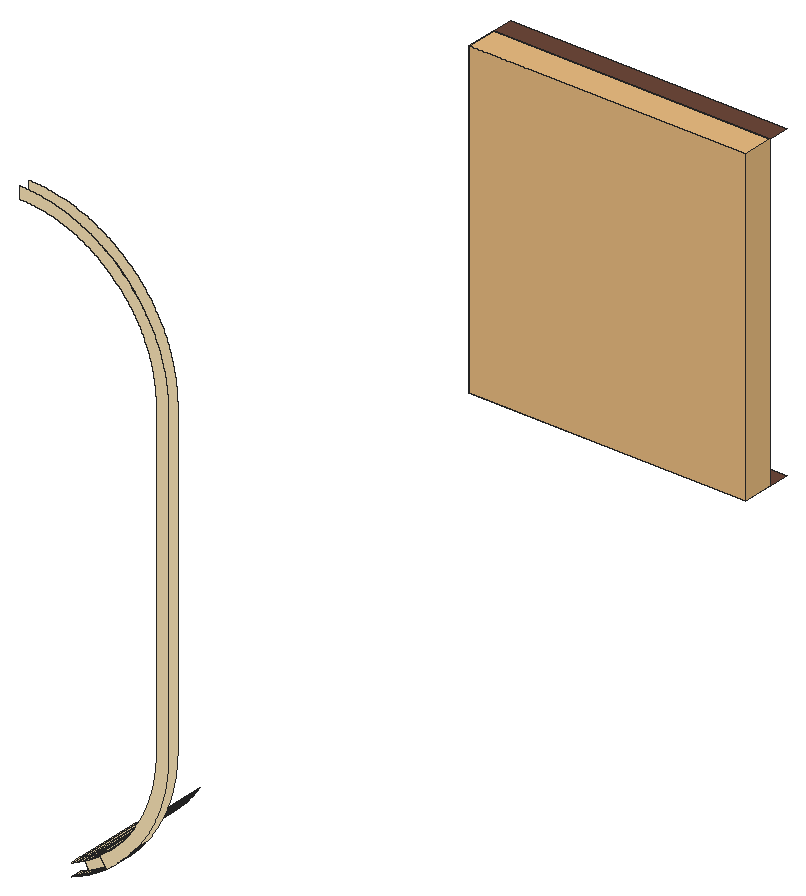
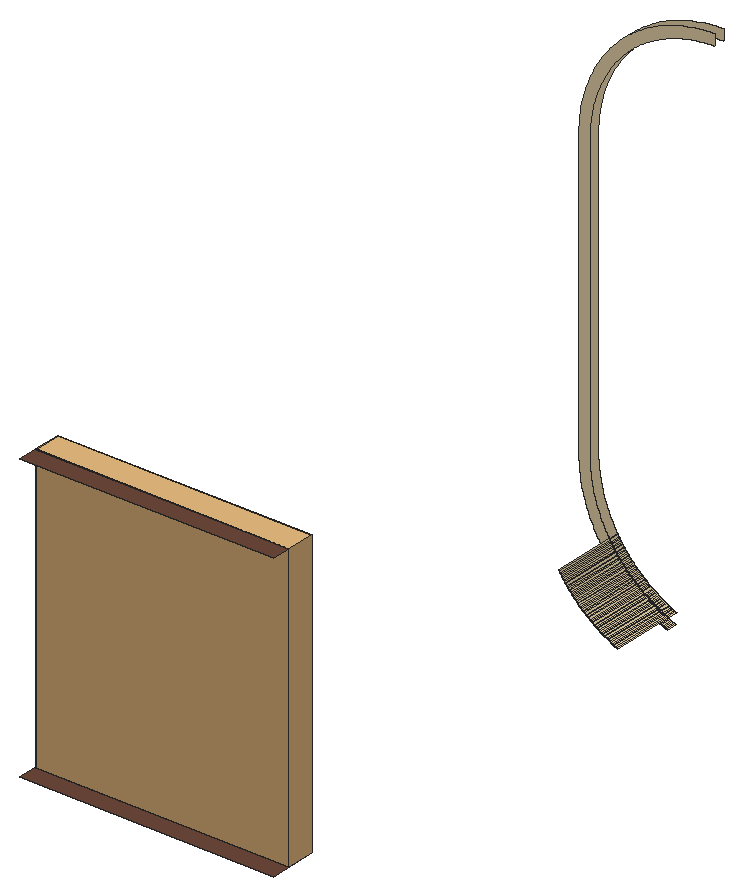
# SketchUp Ruby script. Lengths in inches.
U = 1.inch
M = Sketchup.active_model
def pt(a) = Geom::Point3d.new(a.map { |v| v * U })
def face(e, loops, mat)
  f = e.add_face(loops[0].map { |a| pt(a) })
  loops[1..].each { |l| e.add_face(l.map { |a| pt(a) }).erase! }
  f.material = f.back_material = mat if mat
  f
end
# faces: each face lists its corners as indices into pts; further lists are holes
def faces(e, pts, list, mat = nil) = list.each { |f| face(e, (f[0].is_a?(Array) ? f : [f]).map { |l| l.map { |i| pts[i] } }, mat) }
# xy, xz, yz: faces in a plane at the given z, y or x. An outline is a flat list of corners, or four numbers for a rectangle; further outlines are holes
def ring(l) = l.size == 4 ? [[l[0], l[1]], [l[2], l[1]], [l[2], l[3]], [l[0], l[3]]] : l.each_slice(2).to_a
def flat(e, list, mat, &to3) = list.each { |f| face(e, (f[0].is_a?(Array) ? f : [f]).map { |l| ring(l).map { |u, v| to3.(u, v) } }, mat) }
def xy(e, z, list, mat = nil) = flat(e, list, mat) { |x, y| [x, y, z] }
def xz(e, y, list, mat = nil) = flat(e, list, mat) { |x, z| [x, y, z] }
def yz(e, x, list, mat = nil) = flat(e, list, mat) { |y, z| [x, y, z] }
def lines(e, pts, list) = list.each { |a, b| e.add_line(pt(pts[a]), pt(pts[b])) }
# prism: a flat outline (further loops are holes) pulled along v
def prism(e, loops, v, mat = nil)
  f = face(e, loops, mat); d = Geom::Vector3d.new(v.map { |x| x * U })
  f.pushpull(f.normal.samedirection?(d) ? d.length : -d.length)
end
def box(e, o, s, mat = nil) = prism(e, [[o, [o[0] + s[0], o[1], o[2]], [o[0] + s[0], o[1] + s[1], o[2]], [o[0], o[1] + s[1], o[2]]]], [0, 0, s[2]], mat)
def at(x, y, z, deg = 0) = Geom::Transformation.translation(pt([x, y, z])) * Geom::Transformation.rotation(ORIGIN, Z_AXIS, deg.degrees)
def axes(o, x, y, z) = Geom::Transformation.new([*x, 0, *y, 0, *z, 0, *pt(o).to_a, 1])
def part(name) = M.definitions.add(name)
# library, detail: a bought-in or finely detailed component or shape, given as its bounding box
def library(name, o, s) = part(name).tap { |d| box(d.entities, o, s) }
def detail(e, o, s) = box(e.add_group.entities, o, s)
def put(e, d, t, mat = nil) = e.add_instance(d, t).tap { |i| i.material = mat if mat }
def group(e, t, mat = nil) = e.add_group.tap { |g| g.transformation = t; g.material = mat if mat }.entities
root = M.entities
M.materials.add("1026 AP 7946 SUNNY SIDE UP").color = [254, 231, 186]
M.materials.add("1916 AP K226 Macadamia Cream-N").color = [109, 72, 58]
c1 = library("Glazed double door",[0,0,0],[5.31,78.43,99.16])
xy(root,162,[[141,326,189,335]],"1916 AP K226 Macadamia Cream-N")
xy(root,216,[[141,326,189,335]],"1916 AP K226 Macadamia Cream-N")
xz(root,213.1,[[168.28,146.97,168.49,147.12,168.69,147.27,168.9,147.42,169.3,147.74,169.49,147.9,169.69,148.06,169.89,148.23,170.08,148.4,170.27,148.56,170.46,148.74,170.84,149.08,171.02,149.26,171.2,149.4375,171.38,149.62,171.5625,149.8,171.74,149.98,171.92,150.16,172.26,150.54,172.44,150.73,172.6,150.92,172.77,151.11,172.94,151.31,173.1,151.51,173.26,151.7,173.58,152.1,173.73,152.31,173.88,152.51,174.03,152.72,174.18,152.92,174.48,153.34,174.62,153.56,174.9,153.98,175.03,154.2,175.17,154.42,175.3,154.63,175.56,155.07,175.68,155.3,175.81,155.52,175.93,155.74,176.17,156.2,176.28,156.42,176.61,157.11,176.72,157.35,176.92,157.81,177.12,158.29,177.21,158.52,177.48,159.24,177.56,159.48,177.65,159.72,177.73,159.97,177.81,160.21,177.88,160.45,177.95,160.7,178.02,160.94,178.09,161.1875,178.16,161.44,178.22,161.68,178.4,162.43,178.6,163.43,178.68,163.93,178.72,164.19,178.75,164.4375,178.79,164.69,178.82,164.94,178.85,165.2,178.875,165.45,178.9,165.71,178.92,165.96,178.9375,166.21,178.95,166.47,178.97,166.72,178.98,166.98,178.99,167.23,179,167.49,179,222.51,178.99,222.77,178.98,223.02,178.97,223.28,178.95,223.53,178.9375,223.79,178.92,224.04,178.9,224.29,178.875,224.55,178.85,224.8,178.82,225.06,178.79,225.31,178.75,225.5625,178.72,225.81,178.68,226.07,178.6,226.57,178.4,227.57,178.22,228.32,178.16,228.56,178.09,228.8125,178.02,229.06,177.95,229.3,177.88,229.55,177.81,229.79,177.73,230.03,177.65,230.28,177.56,230.52,177.48,230.76,177.21,231.48,177.12,231.71,176.92,232.19,176.72,232.65,176.61,232.89,176.28,233.58,176.17,233.8,175.93,234.26,175.81,234.48,175.68,234.7,175.56,234.93,175.3,235.37,175.17,235.58,175.03,235.8,174.9,236.02,174.62,236.44,174.48,236.66,174.18,237.08,174.03,237.28,173.88,237.49,173.73,237.69,173.58,237.9,173.26,238.3,173.1,238.49,172.94,238.69,172.77,238.89,172.6,239.08,172.44,239.27,172.26,239.46,171.92,239.84,171.74,240.02,171.5625,240.2,171.38,240.38,171.2,240.5625,171.02,240.74,170.84,240.92,170.46,241.26,170.27,241.44,170.08,241.6,169.89,241.77,169.69,241.94,169.49,242.1,169.3,242.26,168.9,242.58,168.69,242.73,168.49,242.88,168.28,243.03,168.08,243.18,167.66,243.48,167.44,243.62,167.02,243.9,166.8,244.03,166.58,244.17,166.37,244.3,165.93,244.56,165.7,244.68,165.48,244.81,165.26,244.93,164.8,245.17,164.58,245.28,163.89,245.61,163.65,245.72,163.19,245.92,162.71,246.12,162.48,246.21,161.76,246.48,161.52,246.56,161.28,246.65,161.03,246.73,160.79,246.81,160.55,246.88,160.3,246.95,160.06,247.02,159.8125,247.09,159.56,247.16,159.32,247.22,158.57,247.4,157.57,247.6,157.07,247.68,156.81,247.72,156.5625,247.75,156.31,247.79,156.06,247.82,155.8,247.85,155.55,247.875,155.29,247.9,155.04,247.92,154.79,247.9375,154.53,247.95,154.28,247.97,154.02,247.98,153.77,247.99,153.51,248,153.24,248,153.23,246,153.47,246,153.71,245.99,153.94,245.98,154.18,245.97,154.41,245.96,154.65,245.94,154.88,245.93,155.12,245.91,155.35,245.88,155.59,245.86,156.05,245.8,156.29,245.77,156.52,245.74,156.75,245.7,156.99,245.67,157.45,245.58,157.68,245.54,158.14,245.44,158.375,245.39,158.6,245.34,159.29,245.16,159.51,245.1,159.74,245.03,159.97,244.97,160.19,244.9,160.42,244.83,160.64,244.75,160.86,244.68,161.09,244.6,161.31,244.52,161.53,244.43,161.75,244.35,161.97,244.26,162.18,244.17,162.62,243.99,162.83,243.89,163.05,243.8,163.26,243.7,163.47,243.59,163.69,243.49,163.9,243.38,164.11,243.28,164.3125,243.17,164.52,243.05,164.73,242.94,164.93,242.82,165.14,242.71,165.34,242.59,165.54,242.46,165.74,242.34,165.9375,242.21,166.14,242.09,166.33,241.96,166.53,241.82,166.72,241.69,166.92,241.55,167.11,241.42,167.49,241.14,167.67,240.99,167.86,240.85,168.04,240.7,168.23,240.55,168.77,240.1,168.94,239.94,169.12,239.78,169.29,239.625,169.46,239.46,169.8,239.14,170.14,238.8,170.46,238.46,170.625,238.29,170.78,238.12,170.94,237.94,171.1,237.77,171.55,237.23,171.7,237.04,171.85,236.86,171.99,236.67,172.14,236.49,172.42,236.11,172.55,235.92,172.69,235.72,172.82,235.53,172.96,235.33,173.09,235.14,173.21,234.9375,173.34,234.74,173.46,234.54,173.59,234.34,173.71,234.14,173.82,233.93,173.94,233.73,174.05,233.52,174.17,233.3125,174.28,233.11,174.38,232.9,174.49,232.69,174.59,232.47,174.7,232.26,174.8,232.05,174.89,231.83,174.99,231.62,175.17,231.18,175.26,230.97,175.35,230.75,175.43,230.53,175.52,230.31,175.6,230.09,175.68,229.86,175.75,229.64,175.83,229.42,175.9,229.19,175.97,228.97,176.03,228.74,176.1,228.51,176.16,228.29,176.34,227.6,176.39,227.375,176.44,227.14,176.54,226.68,176.58,226.45,176.67,225.99,176.7,225.75,176.74,225.52,176.77,225.29,176.8,225.05,176.86,224.59,176.88,224.35,176.91,224.12,176.93,223.88,176.94,223.65,176.96,223.41,176.97,223.18,176.98,222.94,176.99,222.71,177,222.47,177,167.53,176.99,167.29,176.98,167.06,176.97,166.82,176.96,166.59,176.94,166.35,176.93,166.12,176.91,165.88,176.88,165.65,176.86,165.41,176.8,164.95,176.77,164.71,176.74,164.48,176.7,164.25,176.67,164.01,176.58,163.55,176.54,163.32,176.44,162.86,176.39,162.625,176.34,162.4,176.16,161.71,176.1,161.49,176.03,161.26,175.97,161.03,175.9,160.81,175.83,160.58,175.75,160.36,175.68,160.14,175.6,159.91,175.52,159.69,175.43,159.47,175.35,159.25,175.26,159.03,175.17,158.82,174.99,158.38,174.89,158.17,174.8,157.95,174.7,157.74,174.59,157.53,174.49,157.31,174.38,157.1,174.28,156.89,174.17,156.6875,174.05,156.48,173.94,156.27,173.82,156.07,173.71,155.86,173.59,155.66,173.46,155.46,173.34,155.26,173.21,155.0625,173.09,154.86,172.96,154.67,172.82,154.47,172.69,154.28,172.55,154.08,172.42,153.89,172.14,153.51,171.99,153.33,171.85,153.14,171.7,152.96,171.55,152.77,171.1,152.23,170.94,152.06,170.78,151.88,170.625,151.71,170.46,151.54,170.14,151.2,169.8,150.86,169.46,150.54,169.29,150.375,169.12,150.22,168.94,150.06,168.77,149.9,168.23,149.45,168.04,149.3,167.86,149.15,167.67,149.01,167.49,148.86,167.11,148.58]],"1026 AP 7946 SUNNY SIDE UP")
xz(root,215.1,[[163.65,144.28,162.83,146.11,163.05,146.2,163.26,146.3,163.47,146.41,163.69,146.51,163.9,146.62,164.11,146.72,164.3125,146.83,164.52,146.95,164.73,147.06,164.93,147.18,165.14,147.29,165.34,147.41,165.54,147.54,165.74,147.66,165.9375,147.79,166.14,147.91,166.33,148.04,166.53,148.18,166.72,148.31,166.92,148.45,167.11,148.58,167.49,148.86,167.67,149.01,167.86,149.15,168.04,149.3,168.23,149.45,168.77,149.9,168.94,150.06,169.12,150.22,169.29,150.375,169.46,150.54,169.8,150.86,170.14,151.2,170.46,151.54,170.625,151.71,170.78,151.88,170.94,152.06,171.1,152.23,171.55,152.77,171.7,152.96,171.85,153.14,171.99,153.33,172.14,153.51,172.42,153.89,172.55,154.08,172.69,154.28,172.82,154.47,172.96,154.67,173.09,154.86,173.21,155.0625,173.34,155.26,173.46,155.46,173.59,155.66,173.71,155.86,173.82,156.07,173.94,156.27,174.05,156.48,174.17,156.6875,174.28,156.89,174.38,157.1,174.49,157.31,174.59,157.53,174.7,157.74,174.8,157.95,174.89,158.17,174.99,158.38,175.17,158.82,175.26,159.03,175.35,159.25,175.43,159.47,175.52,159.69,175.6,159.91,175.68,160.14,175.75,160.36,175.83,160.58,175.9,160.81,175.97,161.03,176.03,161.26,176.1,161.49,176.16,161.71,176.34,162.4,176.39,162.625,176.44,162.86,176.54,163.32,176.58,163.55,176.67,164.01,176.7,164.25,176.74,164.48,176.77,164.71,176.8,164.95,176.86,165.41,176.88,165.65,176.91,165.88,176.93,166.12,176.94,166.35,176.96,166.59,176.97,166.82,176.98,167.06,176.99,167.29,177,167.53,177,222.47,176.99,222.71,176.98,222.94,176.97,223.18,176.96,223.41,176.94,223.65,176.93,223.88,176.91,224.12,176.88,224.35,176.86,224.59,176.8,225.05,176.77,225.29,176.74,225.52,176.7,225.75,176.67,225.99,176.58,226.45,176.54,226.68,176.44,227.14,176.39,227.375,176.34,227.6,176.16,228.29,176.1,228.51,176.03,228.74,175.97,228.97,175.9,229.19,175.83,229.42,175.75,229.64,175.68,229.86,175.6,230.09,175.52,230.31,175.43,230.53,175.35,230.75,175.26,230.97,175.17,231.18,174.99,231.62,174.89,231.83,174.8,232.05,174.7,232.26,174.59,232.47,174.49,232.69,174.38,232.9,174.28,233.11,174.17,233.3125,174.05,233.52,173.94,233.73,173.82,233.93,173.71,234.14,173.59,234.34,173.46,234.54,173.34,234.74,173.21,234.9375,173.09,235.14,172.96,235.33,172.82,235.53,172.69,235.72,172.55,235.92,172.42,236.11,172.14,236.49,171.99,236.67,171.85,236.86,171.7,237.04,171.55,237.23,171.1,237.77,170.94,237.94,170.78,238.12,170.625,238.29,170.46,238.46,170.14,238.8,169.8,239.14,169.46,239.46,169.29,239.625,169.12,239.78,168.94,239.94,168.77,240.1,168.23,240.55,168.04,240.7,167.86,240.85,167.67,240.99,167.49,241.14,167.11,241.42,166.92,241.55,166.72,241.69,166.53,241.82,166.33,241.96,166.14,242.09,165.9375,242.21,165.74,242.34,165.54,242.46,165.34,242.59,165.14,242.71,164.93,242.82,164.73,242.94,164.52,243.05,164.3125,243.17,164.11,243.28,163.9,243.38,163.69,243.49,163.47,243.59,163.26,243.7,163.05,243.8,162.83,243.89,162.62,243.99,162.18,244.17,161.97,244.26,161.75,244.35,161.53,244.43,161.31,244.52,161.09,244.6,160.86,244.68,160.64,244.75,160.42,244.83,160.19,244.9,159.97,244.97,159.74,245.03,159.51,245.1,159.29,245.16,158.6,245.34,158.375,245.39,158.14,245.44,157.68,245.54,157.45,245.58,156.99,245.67,156.75,245.7,156.52,245.74,156.29,245.77,156.05,245.8,155.59,245.86,155.35,245.88,155.12,245.91,154.88,245.93,154.65,245.94,154.41,245.96,154.18,245.97,153.94,245.98,153.71,245.99,153.47,246,153.23,246,153.24,248,153.51,248,153.77,247.99,154.02,247.98,154.28,247.97,154.53,247.95,154.79,247.9375,155.04,247.92,155.29,247.9,155.55,247.875,155.8,247.85,156.06,247.82,156.31,247.79,156.5625,247.75,156.81,247.72,157.07,247.68,157.57,247.6,158.57,247.4,159.32,247.22,159.56,247.16,159.8125,247.09,160.06,247.02,160.3,246.95,160.55,246.88,160.79,246.81,161.03,246.73,161.28,246.65,161.52,246.56,161.76,246.48,162.48,246.21,162.71,246.12,163.19,245.92,163.65,245.72,163.89,245.61,164.58,245.28,164.8,245.17,165.26,244.93,165.48,244.81,165.7,244.68,165.93,244.56,166.37,244.3,166.58,244.17,166.8,244.03,167.02,243.9,167.44,243.62,167.66,243.48,168.08,243.18,168.28,243.03,168.49,242.88,168.69,242.73,168.9,242.58,169.3,242.26,169.49,242.1,169.69,241.94,169.89,241.77,170.08,241.6,170.27,241.44,170.46,241.26,170.84,240.92,171.02,240.74,171.2,240.5625,171.38,240.38,171.5625,240.2,171.74,240.02,171.92,239.84,172.26,239.46,172.44,239.27,172.6,239.08,172.77,238.89,172.94,238.69,173.1,238.49,173.26,238.3,173.58,237.9,173.73,237.69,173.88,237.49,174.03,237.28,174.18,237.08,174.48,236.66,174.62,236.44,174.9,236.02,175.03,235.8,175.17,235.58,175.3,235.37,175.56,234.93,175.68,234.7,175.81,234.48,175.93,234.26,176.17,233.8,176.28,233.58,176.61,232.89,176.72,232.65,176.92,232.19,177.12,231.71,177.21,231.48,177.48,230.76,177.56,230.52,177.65,230.28,177.73,230.03,177.81,229.79,177.88,229.55,177.95,229.3,178.02,229.06,178.09,228.8125,178.16,228.56,178.22,228.32,178.4,227.57,178.6,226.57,178.68,226.07,178.72,225.81,178.75,225.5625,178.79,225.31,178.82,225.06,178.85,224.8,178.875,224.55,178.9,224.29,178.92,224.04,178.9375,223.79,178.95,223.53,178.97,223.28,178.98,223.02,178.99,222.77,179,222.51,179,167.49,178.99,167.23,178.98,166.98,178.97,166.72,178.95,166.47,178.9375,166.21,178.92,165.96,178.9,165.71,178.875,165.45,178.85,165.2,178.82,164.94,178.79,164.69,178.75,164.4375,178.72,164.19,178.68,163.93,178.6,163.43,178.4,162.43,178.22,161.68,178.16,161.44,178.09,161.1875,178.02,160.94,177.95,160.7,177.88,160.45,177.81,160.21,177.73,159.97,177.65,159.72,177.56,159.48,177.48,159.24,177.21,158.52,177.12,158.29,176.92,157.81,176.72,157.35,176.61,157.11,176.28,156.42,176.17,156.2,175.93,155.74,175.81,155.52,175.68,155.3,175.56,155.07,175.3,154.63,175.17,154.42,175.03,154.2,174.9,153.98,174.62,153.56,174.48,153.34,174.18,152.92,174.03,152.72,173.88,152.51,173.73,152.31,173.58,152.1,173.26,151.7,173.1,151.51,172.94,151.31,172.77,151.11,172.6,150.92,172.44,150.73,172.26,150.54,171.92,150.16,171.74,149.98,171.5625,149.8,171.38,149.62,171.2,149.4375,171.02,149.26,170.84,149.08,170.46,148.74,170.27,148.56,170.08,148.4,169.89,148.23,169.69,148.06,169.49,147.9,169.3,147.74,168.9,147.42,168.69,147.27,168.49,147.12,168.28,146.97,168.08,146.82,167.66,146.52,167.44,146.38,167.02,146.1,166.8,145.97,166.58,145.83,166.37,145.7,165.93,145.44,165.7,145.32,165.48,145.19,165.26,145.07,164.8,144.83,164.58,144.72,163.89,144.39]],"1026 AP 7946 SUNNY SIDE UP")
p = [[162.24,213.1,143.7],[162.24,215.1,143.7],[162.48,215.1,143.79],[162.48,213.1,143.79],[162.71,215.1,143.88],[162.71,213.1,143.88],
  [162.95,215.1,143.98],[162.95,213.1,143.98],[163.19,215.1,144.08],[163.19,213.1,144.08],[163.42,215.1,144.18],[163.42,213.1,144.18],
  [163.65,215.1,144.28],[163.65,213.1,144.28],[163.89,215.1,144.39],[163.89,213.1,144.39],[164.12,215.1,144.5],[164.12,213.1,144.5],
  [164.35,215.1,144.61],[164.35,213.1,144.61],[164.58,215.1,144.72],[164.58,213.1,144.72],[164.8,215.1,144.83],[164.8,213.1,144.83],
  [165.03,215.1,144.95],[165.03,213.1,144.95],[165.26,215.1,145.07],[165.26,213.1,145.07],[165.48,215.1,145.19],[165.48,213.1,145.19],
  [165.7,215.1,145.32],[165.7,213.1,145.32],[165.93,215.1,145.44],[165.93,213.1,145.44],[166.15,215.1,145.57],[166.15,213.1,145.57],
  [166.37,215.1,145.7],[166.37,213.1,145.7],[166.58,215.1,145.83],[166.58,213.1,145.83],[162.4,213.1,145.92],[162.4,215,145.92],
  [162.18,215,145.83],[162.18,213.1,145.83],[166.8,215.1,145.97],[166.8,213.1,145.97],[162.18,215.1,145.83],[162.4,215.1,145.92],
  [162.18,227,145.83],[162.4,227,145.92],[162.62,213.1,146.01],[162.62,215,146.01],[162.62,215.1,146.01],[162.62,227,146.01],
  [162.83,213.1,146.11],[162.83,215,146.11],[167.02,215.1,146.1],[167.02,213.1,146.1],[162.83,215.1,146.11],[162.83,227,146.11],
  [163.05,213.1,146.2],[163.05,215,146.2],[167.23,215.1,146.24],[167.23,213.1,146.24],[163.05,215.1,146.2],[163.05,227,146.2],
  [163.26,213.1,146.3],[163.26,215,146.3],[167.44,215.1,146.38],[167.44,213.1,146.38],[163.26,215.1,146.3],[163.26,227,146.3],
  [163.47,213.1,146.41],[163.47,215,146.41],[163.47,215.1,146.41],[163.47,227,146.41],[163.69,213.1,146.51],[163.69,215,146.51],
  [167.66,215.1,146.52],[167.66,213.1,146.52],[163.69,215.1,146.51],[163.69,227,146.51],[163.9,213.1,146.62],[163.9,215,146.62],
  [167.87,215.1,146.67],[167.87,213.1,146.67],[163.9,215.1,146.62],[163.9,227,146.62],[164.11,213.1,146.72],[164.11,215,146.72],
  [164.11,215.1,146.72],[164.11,227,146.72],[164.3125,213.1,146.83],[164.3125,215,146.83],[168.08,215.1,146.82],[168.08,213.1,146.82],
  [164.3125,215.1,146.83],[164.3125,227,146.83],[164.52,213.1,146.95],[164.52,215,146.95],[168.28,215.1,146.97],[168.28,213.1,146.97],
  [164.52,215.1,146.95],[164.52,227,146.95],[164.73,213.1,147.06],[164.73,215,147.06],[164.73,215.1,147.06],[164.73,227,147.06],
  [168.49,215.1,147.12],[168.49,213.1,147.12],[164.93,213.1,147.18],[164.93,215,147.18],[168.69,215.1,147.27],[168.69,213.1,147.27],
  [164.93,215.1,147.18],[164.93,227,147.18],[165.14,213.1,147.29],[165.14,215,147.29],[165.14,215.1,147.29],[165.14,227,147.29],
  [165.34,213.1,147.41],[165.34,215,147.41],[168.9,215.1,147.42],[168.9,213.1,147.42],[165.34,215.1,147.41],[165.34,227,147.41],
  [165.54,213.1,147.54],[165.54,215,147.54],[169.1,215.1,147.58],[169.1,213.1,147.58],[165.54,215.1,147.54],[165.54,227,147.54],
  [165.74,213.1,147.66],[165.74,215,147.66],[165.74,215.1,147.66],[165.74,227,147.66],[169.3,215.1,147.74],[169.3,213.1,147.74],
  [165.9375,213.1,147.79],[165.9375,215,147.79],[169.49,215.1,147.9],[169.49,213.1,147.9],[165.9375,215.1,147.79],[165.9375,227,147.79],
  [166.14,213.1,147.91],[166.14,215,147.91],[166.14,215.1,147.91],[166.14,227,147.91],[166.33,213.1,148.04],[166.33,215,148.04],
  [169.69,215.1,148.06],[169.69,213.1,148.06],[166.33,215.1,148.04],[166.33,227,148.04],[166.53,213.1,148.18],[166.53,215,148.18],
  [166.53,215.1,148.18],[166.53,227,148.18],[169.89,215.1,148.23],[169.89,213.1,148.23],[166.72,213.1,148.31],[166.72,215,148.31],
  [170.08,215.1,148.4],[170.08,213.1,148.4],[166.72,215.1,148.31],[166.72,227,148.31],[166.92,213.1,148.45],[166.92,215,148.45],
  [166.92,215.1,148.45],[166.92,227,148.45],[167.11,213.1,148.58],[167.11,215,148.58],[170.27,215.1,148.56],[170.27,213.1,148.56],
  [167.11,215.1,148.58],[167.11,227,148.58],[167.3,213.1,148.72],[167.3,215,148.72],[170.46,215.1,148.74],[170.46,213.1,148.74],
  [167.3,215.1,148.72],[167.3,227,148.72],[167.49,213.1,148.86],[167.49,215,148.86],[170.65,215.1,148.91],[170.65,213.1,148.91],
  [167.49,215.1,148.86],[167.49,227,148.86],[167.67,213.1,149.01],[167.67,215,149.01],[170.84,215.1,149.08],[170.84,213.1,149.08],
  [167.67,215.1,149.01],[167.67,227,149.01],[167.86,213.1,149.15],[167.86,215,149.15],[167.86,215.1,149.15],[167.86,227,149.15],
  [171.02,215.1,149.26],[171.02,213.1,149.26],[168.04,213.1,149.3],[168.04,215,149.3],[168.04,215.1,149.3],[168.04,227,149.3],
  [168.23,213.1,149.45],[168.23,215,149.45],[171.2,215.1,149.4375],[171.2,213.1,149.4375],[168.23,215.1,149.45],[168.23,227,149.45],
  [168.41,213.1,149.6],[168.41,215,149.6],[171.38,215.1,149.62],[171.38,213.1,149.62],[168.41,215.1,149.6],[168.41,227,149.6],
  [168.59,213.1,149.75],[168.59,215,149.75],[171.5625,215.1,149.8],[171.5625,213.1,149.8],[168.59,215.1,149.75],[168.59,227,149.75],
  [168.77,213.1,149.9],[168.77,215,149.9],[171.74,215.1,149.98],[171.74,213.1,149.98],[168.77,215.1,149.9],[168.77,227,149.9],
  [168.94,213.1,150.06],[168.94,215,150.06],[168.94,215.1,150.06],[168.94,227,150.06],[171.92,215.1,150.16],[171.92,213.1,150.16],
  [169.12,213.1,150.22],[169.12,215,150.22],[169.12,215.1,150.22],[169.12,227,150.22],[169.29,213.1,150.375],[169.29,215,150.375],
  [172.09,215.1,150.35],[172.09,213.1,150.35],[169.29,215.1,150.375],[169.29,227,150.375],[169.46,213.1,150.54],[169.46,215,150.54],
  [172.26,215.1,150.54],[172.26,213.1,150.54],[169.46,215.1,150.54],[169.46,227,150.54],[169.63,213.1,150.7],[169.63,215,150.7],
  [172.44,215.1,150.73],[172.44,213.1,150.73],[169.63,215.1,150.7],[169.63,227,150.7],[169.8,213.1,150.86],[169.8,215,150.86],
  [172.6,215.1,150.92],[172.6,213.1,150.92],[169.8,215.1,150.86],[169.8,227,150.86],[169.97,213.1,151.03],[169.97,215,151.03],
  [172.77,215.1,151.11],[172.77,213.1,151.11],[169.97,215.1,151.03],[169.97,227,151.03],[170.14,213.1,151.2],[170.14,215,151.2],
  [170.14,215.1,151.2],[170.14,227,151.2],[172.94,215.1,151.31],[172.94,213.1,151.31],[170.3,213.1,151.37],[170.3,215,151.37],
  [170.3,215.1,151.37],[170.3,227,151.37],[173.1,215.1,151.51],[173.1,213.1,151.51],[170.46,213.1,151.54],[170.46,215,151.54],
  [170.46,215.1,151.54],[170.46,227,151.54],[170.625,213.1,151.71],[170.625,215,151.71],[173.26,215.1,151.7],[173.26,213.1,151.7],
  [170.625,215.1,151.71],[170.625,227,151.71],[170.78,213.1,151.88],[170.78,215,151.88],[173.42,215.1,151.9],[173.42,213.1,151.9],
  [170.78,215.1,151.88],[170.78,227,151.88],[170.94,213.1,152.06],[170.94,215,152.06],[170.94,215.1,152.06],[170.94,227,152.06],
  [171.1,213.1,152.23],[171.1,215,152.23],[171.1,215.1,152.23],[171.1,227,152.23],[171.25,213.1,152.41],[171.25,215,152.41],
  [171.25,215.1,152.41],[171.25,227,152.41],[171.4,213.1,152.59],[171.4,215,152.59],[171.4,215.1,152.59],[171.4,227,152.59],
  [171.55,213.1,152.77],[171.55,215,152.77],[171.55,215.1,152.77],[171.55,227,152.77],[171.7,213.1,152.96],[171.7,215,152.96],
  [171.7,215.1,152.96],[171.7,227,152.96],[171.85,213.1,153.14],[171.85,215,153.14],[171.85,215.1,153.14],[171.85,227,153.14],
  [171.99,213.1,153.33],[171.99,215,153.33],[171.99,215.1,153.33],[171.99,227,153.33],[172.14,213.1,153.51],[172.14,215,153.51],
  [172.14,215.1,153.51],[172.14,227,153.51],[172.28,213.1,153.7],[172.28,215,153.7],[172.28,215.1,153.7],[172.28,227,153.7],
  [172.42,213.1,153.89],[172.42,215,153.89],[172.42,215.1,153.89],[172.42,227,153.89],[172.55,213.1,154.08],[172.55,215,154.08],
  [172.55,215.1,154.08],[172.55,227,154.08],[172.69,213.1,154.28],[172.69,215,154.28],[172.69,215.1,154.28],[172.69,227,154.28],
  [172.82,213.1,154.47],[172.82,215,154.47],[172.82,215.1,154.47],[172.82,227,154.47],[172.96,213.1,154.67],[172.96,215,154.67],
  [172.96,215.1,154.67],[172.96,227,154.67],[173.09,213.1,154.86],[173.09,215,154.86],[173.09,215.1,154.86],[173.09,227,154.86],
  [173.21,213.1,155.0625],[173.21,215,155.0625],[173.21,215.1,155.0625],[173.21,227,155.0625],[173.34,213.1,155.26],[173.34,215,155.26],
  [173.34,215.1,155.26],[173.34,227,155.26],[173.46,215,155.46],[173.46,215.1,155.46]]
faces(root,p,[[0,1,2,3],[3,2,4,5],[5,4,6,7],[7,6,8,9],[9,8,10,11],[11,10,12,13],[13,12,14,15],[15,14,16,17],
  [17,16,18,19],[19,18,20,21],[21,20,22,23],[23,22,24,25],[25,24,26,27],[27,26,28,29],[29,28,30,31],[31,30,32,33],
  [33,32,34,35],[35,34,36,37],[37,36,38,39],[40,41,42,43],[39,38,44,45],[46,42,41,47],[48,46,47,49],[50,51,41,40],
  [47,41,51,52],[49,47,52,53],[54,55,51,50],[45,44,56,57],[52,51,55,58],[53,52,58,59],[60,61,55,54],[57,56,62,63],
  [58,55,61,64],[59,58,64,65],[66,67,61,60],[63,62,68,69],[64,61,67,70],[65,64,70,71],[72,73,67,66],[70,67,73,74],
  [71,70,74,75],[76,77,73,72],[69,68,78,79],[74,73,77,80],[75,74,80,81],[82,83,77,76],[79,78,84,85],[80,77,83,86],
  [81,80,86,87],[88,89,83,82],[86,83,89,90],[87,86,90,91],[92,93,89,88],[85,84,94,95],[90,89,93,96],[91,90,96,97],
  [98,99,93,92],[95,94,100,101],[96,93,99,102],[97,96,102,103],[104,105,99,98],[102,99,105,106],[103,102,106,107],[101,100,108,109],
  [110,111,105,104],[109,108,112,113],[106,105,111,114],[107,106,114,115],[116,117,111,110],[114,111,117,118],[115,114,118,119],[120,121,117,116],
  [113,112,122,123],[118,117,121,124],[119,118,124,125],[126,127,121,120],[123,122,128,129],[124,121,127,130],[125,124,130,131],[132,133,127,126],
  [130,127,133,134],[131,130,134,135],[129,128,136,137],[138,139,133,132],[137,136,140,141],[134,133,139,142],[135,134,142,143],[144,145,139,138],
  [142,139,145,146],[143,142,146,147],[148,149,145,144],[141,140,150,151],[146,145,149,152],[147,146,152,153],[154,155,149,148],[152,149,155,156],
  [153,152,156,157],[151,150,158,159],[160,161,155,154],[159,158,162,163],[156,155,161,164],[157,156,164,165],[166,167,161,160],[164,161,167,168],
  [165,164,168,169],[170,171,167,166],[163,162,172,173],[168,167,171,174],[169,168,174,175],[176,177,171,170],[173,172,178,179],[174,171,177,180],
  [175,174,180,181],[182,183,177,176],[179,178,184,185],[180,177,183,186],[181,180,186,187],[188,189,183,182],[185,184,190,191],[186,183,189,192],
  [187,186,192,193],[194,195,189,188],[192,189,195,196],[193,192,196,197],[191,190,198,199],[200,201,195,194],[196,195,201,202],[197,196,202,203],
  [204,205,201,200],[199,198,206,207],[202,201,205,208],[203,202,208,209],[210,211,205,204],[207,206,212,213],[208,205,211,214],[209,208,214,215],
  [216,217,211,210],[213,212,218,219],[214,211,217,220],[215,214,220,221],[222,223,217,216],[219,218,224,225],[220,217,223,226],[221,220,226,227],
  [228,229,223,222],[226,223,229,230],[227,226,230,231],[225,224,232,233],[234,235,229,228],[230,229,235,236],[231,230,236,237],[238,239,235,234],
  [233,232,240,241],[236,235,239,242],[237,236,242,243],[244,245,239,238],[241,240,246,247],[242,239,245,248],[243,242,248,249],[250,251,245,244],
  [247,246,252,253],[248,245,251,254],[249,248,254,255],[256,257,251,250],[253,252,258,259],[254,251,257,260],[255,254,260,261],[262,263,257,256],
  [259,258,264,265],[260,257,263,266],[261,260,266,267],[268,269,263,262],[266,263,269,270],[267,266,270,271],[265,264,272,273],[274,275,269,268],
  [270,269,275,276],[271,270,276,277],[273,272,278,279],[280,281,275,274],[276,275,281,282],[277,276,282,283],[284,285,281,280],[279,278,286,287],
  [282,281,285,288],[283,282,288,289],[290,291,285,284],[287,286,292,293],[288,285,291,294],[289,288,294,295],[296,297,291,290],[294,291,297,298],
  [295,294,298,299],[300,301,297,296],[298,297,301,302],[299,298,302,303],[304,305,301,300],[302,301,305,306],[303,302,306,307],[308,309,305,304],
  [306,305,309,310],[307,306,310,311],[312,313,309,308],[310,309,313,314],[311,310,314,315],[316,317,313,312],[314,313,317,318],[315,314,318,319],
  [320,321,317,316],[318,317,321,322],[319,318,322,323],[324,325,321,320],[322,321,325,326],[323,322,326,327],[328,329,325,324],[326,325,329,330],
  [327,326,330,331],[332,333,329,328],[330,329,333,334],[331,330,334,335],[336,337,333,332],[334,333,337,338],[335,334,338,339],[340,341,337,336],
  [338,337,341,342],[339,338,342,343],[344,345,341,340],[342,341,345,346],[343,342,346,347],[348,349,345,344],[346,345,349,350],[347,346,350,351],
  [352,353,349,348],[350,349,353,354],[351,350,354,355],[356,357,353,352],[354,353,357,358],[355,354,358,359],[360,361,357,356],[358,357,361,362],
  [359,358,362,363],[364,365,361,360],[362,361,365,366],[363,362,366,367],[366,365,368,369]],"1026 AP 7946 SUNNY SIDE UP")
put(root,c1,axes([141,331.31,162],[0,-1,0],[0.61205,0,0],[0,0,0.54459]),"1026 AP 7946 SUNNY SIDE UP")
